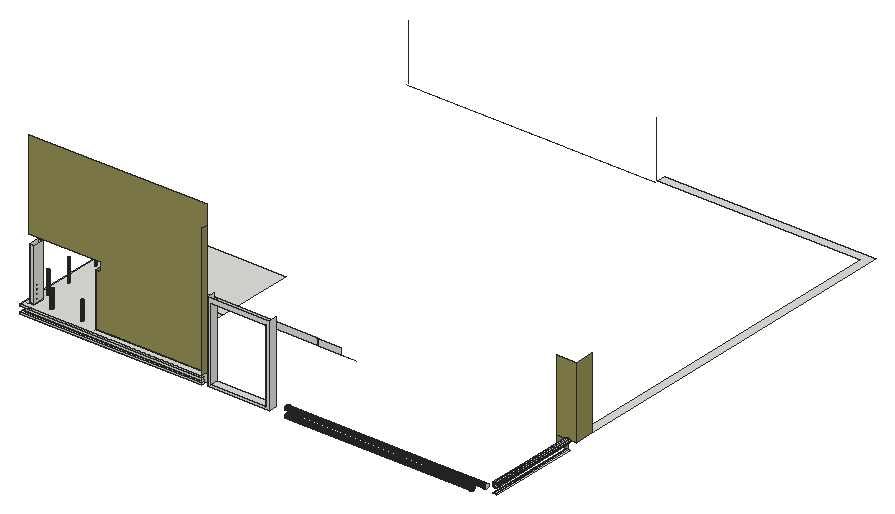
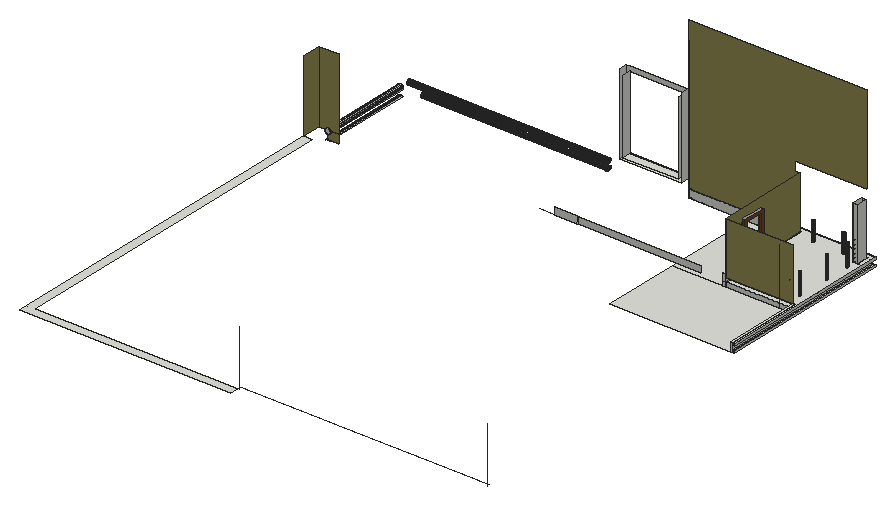
# SketchUp Ruby script. Lengths in inches.
U = 1.inch
M = Sketchup.active_model
def pt(a) = Geom::Point3d.new(a.map { |v| v * U })
def face(e, loops, mat)
  f = e.add_face(loops[0].map { |a| pt(a) })
  loops[1..].each { |l| e.add_face(l.map { |a| pt(a) }).erase! }
  f.material = f.back_material = mat if mat
  f
end
# faces: each face lists its corners as indices into pts; further lists are holes
def faces(e, pts, list, mat = nil) = list.each { |f| face(e, (f[0].is_a?(Array) ? f : [f]).map { |l| l.map { |i| pts[i] } }, mat) }
# xy, xz, yz: faces in a plane at the given z, y or x. An outline is a flat list of corners, or four numbers for a rectangle; further outlines are holes
def ring(l) = l.size == 4 ? [[l[0], l[1]], [l[2], l[1]], [l[2], l[3]], [l[0], l[3]]] : l.each_slice(2).to_a
def flat(e, list, mat, &to3) = list.each { |f| face(e, (f[0].is_a?(Array) ? f : [f]).map { |l| ring(l).map { |u, v| to3.(u, v) } }, mat) }
def xy(e, z, list, mat = nil) = flat(e, list, mat) { |x, y| [x, y, z] }
def xz(e, y, list, mat = nil) = flat(e, list, mat) { |x, z| [x, y, z] }
def yz(e, x, list, mat = nil) = flat(e, list, mat) { |y, z| [x, y, z] }
def lines(e, pts, list) = list.each { |a, b| e.add_line(pt(pts[a]), pt(pts[b])) }
# prism: a flat outline (further loops are holes) pulled along v
def prism(e, loops, v, mat = nil)
  f = face(e, loops, mat); d = Geom::Vector3d.new(v.map { |x| x * U })
  f.pushpull(f.normal.samedirection?(d) ? d.length : -d.length)
end
def box(e, o, s, mat = nil) = prism(e, [[o, [o[0] + s[0], o[1], o[2]], [o[0] + s[0], o[1] + s[1], o[2]], [o[0], o[1] + s[1], o[2]]]], [0, 0, s[2]], mat)
def at(x, y, z, deg = 0) = Geom::Transformation.translation(pt([x, y, z])) * Geom::Transformation.rotation(ORIGIN, Z_AXIS, deg.degrees)
def axes(o, x, y, z) = Geom::Transformation.new([*x, 0, *y, 0, *z, 0, *pt(o).to_a, 1])
def part(name) = M.definitions.add(name)
# library, detail: a bought-in or finely detailed component or shape, given as its bounding box
def library(name, o, s) = part(name).tap { |d| box(d.entities, o, s) }
def detail(e, o, s) = box(e.add_group.entities, o, s)
def put(e, d, t, mat = nil) = e.add_instance(d, t).tap { |i| i.material = mat if mat }
def group(e, t, mat = nil) = e.add_group.tap { |g| g.transformation = t; g.material = mat if mat }.entities
root = M.entities
M.materials.add("[0057_DarkKhaki]").color = [150, 145, 85]
M.materials.add("[0137_Black]").color = [71, 71, 71]
M.materials.add("[Wood Veneer 01]").color = [120, 70, 37]
xy(root,417.65,[[11.875,15.1875,200.79,18.1875],[8.875,18.1875,11.875,116.75],[11.875,18.1875,139.9375,116.75],[8.875,116.75,9.8125,199.5],[9.8125,116.75,11.875,199.5],
  [11.875,116.75,139.9375,199.5]])
xy(root,417.72,[[7.3125,12.1875,7.3125,199.5,9.8125,199.5,9.8125,15.1875,82.85,15.1875,82.85,12.1875],[82.85,12.1875,200.79,15.1875],[9.8125,15.1875,9.8125,116.75,11.875,116.75,11.875,18.1875,82.85,18.1875,82.85,15.1875],[82.85,15.1875,200.79,18.1875],[11.875,18.1875,12.375,21.1875],
  [12.375,18.1875,82.85,21.1875],[11.875,21.1875,12.375,21.75],[12.375,21.1875,82.85,21.75],[11.875,21.75,12.375,116.75],[12.375,21.75,82.85,116.75]])
xy(root,419.53,[[7.3125,12.1875,200.79,12.1875,200.79,15.1875,9.8125,15.1875,9.8125,199.5,7.3125,199.5]])
xy(root,422.78,[[11.875,21.1875,12.375,116.75],[12.375,21.1875,82.85,116.75]])
xy(root,423,[[501.6875,143.77,510.6875,143.77,510.6875,520.875,286.17,520.875,286.17,511.875,501.6875,511.875]])
xy(root,424.77,[[7.1875,12.1875,7.1875,199.5,9.8125,199.5,9.8125,15.1875,200.79,15.1875,200.79,12.1875]])
xy(root,425.13,[[213.98,3.1875,279.92,12.1875]])
xy(root,426.78,[[[7.1875,12.1875,7.1875,199.5,9.8125,199.5,9.8125,116.75,82.85,116.75,82.85,95.21,79.85,95.21,79.85,92.21,82.85,92.21,82.85,73.09,79.85,73.09,79.85,70.09,82.85,70.09,82.85,18.1875,200.79,18.1875,200.79,12.1875,16.875,12.1875,16.875,30.25,9.8125,30.25,9.8125,18.1875,11.9375,18.1875,11.9375,19,16.875,19,16.875,12.1875],[64.82,21.64,65.21,21.69,65.57,21.84,65.88,22.08,66.12,22.39,66.27,22.75,66.32,23.14,66.27,23.53,66.12,23.89,65.88,24.2,65.57,24.44,65.21,24.59,64.82,24.64,64.43,24.59,64.07,24.44,63.76,24.2,63.52,23.89,63.375,23.53,63.32,23.14,63.375,22.75,63.52,22.39,63.76,22.08,64.07,21.84,64.43,21.69],[32.63,21.64,33.02,21.69,33.38,21.84,33.7,22.08,33.93,22.39,34.08,22.75,34.13,23.14,34.08,23.53,33.93,23.89,33.7,24.2,33.38,24.44,33.02,24.59,32.63,24.64,32.25,24.59,31.88,24.44,31.57,24.2,31.34,23.89,31.1875,23.53,31.13,23.14,31.1875,22.75,31.34,22.39,31.57,22.08,31.88,21.84,32.25,21.69],[15.22,38.96,15.47,39,15.69,39.09,15.88,39.24,16.03,39.43,16.125,39.65,16.15,39.89,16.125,40.14,16.03,40.36,15.88,40.55,15.69,40.7,15.47,40.79,15.22,40.82,14.98,40.79,14.76,40.7,14.57,40.55,14.42,40.36,14.33,40.14,14.29,39.89,14.33,39.65,14.42,39.43,14.57,39.24,14.76,39.09,14.98,39],[15.85,101.9,16.09,101.93,16.31,102.03,16.51,102.17,16.66,102.37,16.75,102.59,16.78,102.83,16.75,103.07,16.66,103.3,16.51,103.49,16.31,103.64,16.09,103.73,15.85,103.76,15.61,103.73,15.38,103.64,15.19,103.49,15.04,103.3,14.95,103.07,14.92,102.83,14.95,102.59,15.04,102.37,15.19,102.17,15.38,102.03,15.61,101.93],[15.85,65.84,16.09,65.87,16.31,65.96,16.51,66.11,16.66,66.3,16.75,66.53,16.78,66.77,16.75,67.01,16.66,67.23,16.51,67.43,16.31,67.58,16.09,67.67,15.85,67.7,15.61,67.67,15.38,67.58,15.19,67.43,15.04,67.23,14.95,67.01,14.92,66.77,14.95,66.53,15.04,66.3,15.19,66.11,15.38,65.96,15.61,65.87]],[9.8125,18.1875,11.9375,30.25],[11.9375,19,16.875,30.25],[79.85,70.09,82.85,73.09],[79.85,92.21,82.85,95.21],
  [9.8125,116.75,11.875,199.5]])
xy(root,426.9,[[[7.1875,12.1875,200.79,12.1875,200.79,18.1875,82.85,18.1875,82.85,70.09,79.85,70.09,79.85,73.09,82.85,73.09,82.85,92.21,79.85,92.21,79.85,95.21,82.85,95.21,82.85,116.75,9.8125,116.75,9.8125,199.5,7.1875,199.5],[11.9375,19,16.875,30.25],[64.82,21.64,64.43,21.69,64.07,21.84,63.76,22.08,63.52,22.39,63.375,22.75,63.32,23.14,63.375,23.53,63.52,23.89,63.76,24.2,64.07,24.44,64.43,24.59,64.82,24.64,65.21,24.59,65.57,24.44,65.88,24.2,66.12,23.89,66.27,23.53,66.32,23.14,66.27,22.75,66.12,22.39,65.88,22.08,65.57,21.84,65.21,21.69],[32.63,21.64,32.25,21.69,31.88,21.84,31.57,22.08,31.34,22.39,31.1875,22.75,31.13,23.14,31.1875,23.53,31.34,23.89,31.57,24.2,31.88,24.44,32.25,24.59,32.63,24.64,33.02,24.59,33.38,24.44,33.7,24.2,33.93,23.89,34.08,23.53,34.13,23.14,34.08,22.75,33.93,22.39,33.7,22.08,33.38,21.84,33.02,21.69],[15.22,38.96,14.98,39,14.76,39.09,14.57,39.24,14.42,39.43,14.33,39.65,14.29,39.89,14.33,40.14,14.42,40.36,14.57,40.55,14.76,40.7,14.98,40.79,15.22,40.82,15.47,40.79,15.69,40.7,15.88,40.55,16.03,40.36,16.125,40.14,16.15,39.89,16.125,39.65,16.03,39.43,15.88,39.24,15.69,39.09,15.47,39],[15.85,101.9,15.61,101.93,15.38,102.03,15.19,102.17,15.04,102.37,14.95,102.59,14.92,102.83,14.95,103.07,15.04,103.3,15.19,103.49,15.38,103.64,15.61,103.73,15.85,103.76,16.09,103.73,16.31,103.64,16.51,103.49,16.66,103.3,16.75,103.07,16.78,102.83,16.75,102.59,16.66,102.37,16.51,102.17,16.31,102.03,16.09,101.93],[15.85,65.84,15.61,65.87,15.38,65.96,15.19,66.11,15.04,66.3,14.95,66.53,14.92,66.77,14.95,67.01,15.04,67.23,15.19,67.43,15.38,67.58,15.61,67.67,15.85,67.7,16.09,67.67,16.31,67.58,16.51,67.43,16.66,67.23,16.75,67.01,16.78,66.77,16.75,66.53,16.66,66.3,16.51,66.11,16.31,65.96,16.09,65.87]]])
xy(root,427.53,[[217.11,3.1875,275.76,12.1875]])
xz(root,3.1875,[[[213.98,425.13,279.92,425.13,279.92,510.53,275.76,510.53,275.76,510.5,213.98,510.5],[217.11,427.53,275.76,505.68]]])
xz(root,12.1875,[[7.3125,417.72,200.79,419.53],[7.1875,424.77,200.79,426.78],[7.1875,426.78,16.875,426.9],[16.875,426.78,200.79,426.9]])
xz(root,15.1875,[[9.8125,417.72,200.79,419.53],[9.8125,419.53,200.79,424.77]])
xz(root,18.1875,[[11.875,417.65,200.79,417.72],[82.85,417.72,200.79,426.78],[82.85,426.78,200.79,426.9]])
xz(root,18.1875,[[82.85,426.9,200.79,426.9,200.79,587.24,11.875,587.24,11.875,493.0625,88.41,493.0625,88.41,483,82.85,483]],"[0057_DarkKhaki]")
xz(root,19,[[11.9375,426.78,16.875,426.9],[11.9375,426.9,16.875,483]])
xz(root,21.1875,[[11.875,417.72,12.375,422.78],[12.375,417.72,82.85,422.78]])
xz(root,30.25,[[11.9375,426.78,16.875,426.9],[[11.9375,426.9,16.875,483],[14.9,434.22,15.21,434.26,15.5,434.375,15.74,434.5625,15.93,434.81,16.05,435.1,16.09,435.4,16.05,435.71,15.93,436,15.74,436.24,15.5,436.43,15.21,436.55,14.9,436.59,14.6,436.55,14.3125,436.43,14.07,436.24,13.875,436,13.76,435.71,13.72,435.4,13.76,435.1,13.875,434.81,14.07,434.5625,14.3125,434.375,14.6,434.26],[14.9,438.47,15.21,438.51,15.5,438.625,15.74,438.8125,15.93,439.06,16.05,439.35,16.09,439.65,16.05,439.96,15.93,440.25,15.74,440.49,15.5,440.68,15.21,440.8,14.9,440.84,14.6,440.8,14.3125,440.68,14.07,440.49,13.875,440.25,13.76,439.96,13.72,439.65,13.76,439.35,13.875,439.06,14.07,438.8125,14.3125,438.625,14.6,438.51],[14.9,442.72,15.21,442.76,15.5,442.875,15.74,443.0625,15.93,443.31,16.05,443.6,16.09,443.9,16.05,444.21,15.93,444.5,15.74,444.74,15.5,444.93,15.21,445.05,14.9,445.09,14.6,445.05,14.3125,444.93,14.07,444.74,13.875,444.5,13.76,444.21,13.72,443.9,13.76,443.6,13.875,443.31,14.07,443.0625,14.3125,442.875,14.6,442.76],[14.9,446.97,15.21,447.01,15.5,447.125,15.74,447.3125,15.93,447.56,16.05,447.85,16.09,448.15,16.05,448.46,15.93,448.75,15.74,448.99,15.5,449.18,15.21,449.3,14.9,449.34,14.6,449.3,14.3125,449.18,14.07,448.99,13.875,448.75,13.76,448.46,13.72,448.15,13.76,447.85,13.875,447.56,14.07,447.3125,14.3125,447.125,14.6,447.01],[14.9,429.97,15.21,430.01,15.5,430.125,15.74,430.3125,15.93,430.56,16.05,430.85,16.09,431.15,16.05,431.46,15.93,431.75,15.74,431.99,15.5,432.18,15.21,432.3,14.9,432.34,14.6,432.3,14.3125,432.18,14.07,431.99,13.875,431.75,13.76,431.46,13.72,431.15,13.76,430.85,13.875,430.56,14.07,430.3125,14.3125,430.125,14.6,430.01]]])
xz(root,70.09,[[79.85,426.78,82.85,426.9]])
xz(root,70.09,[[79.85,426.9,82.85,473.09]],"[Wood Veneer 01]")
xz(root,73.09,[[79.85,426.78,82.85,426.9]])
xz(root,73.09,[[79.85,426.9,82.85,470.09]],"[Wood Veneer 01]")
xz(root,92.21,[[79.85,426.78,82.85,426.9]])
xz(root,92.21,[[79.85,426.9,82.85,470.09]],"[Wood Veneer 01]")
xz(root,95.21,[[79.85,426.78,82.85,426.9]])
xz(root,95.21,[[79.85,426.9,82.85,473.09]],"[Wood Veneer 01]")
xz(root,116.75,[[9.8125,417.65,11.875,417.72],[82.85,417.65,86.03,423],[11.875,417.72,12.375,422.78],[12.375,417.72,82.85,422.78],[82.85,423,86.03,429.99],
  [9.8125,426.78,11.875,426.9],[11.875,426.78,82.85,426.9]])
xz(root,116.75,[[[11.875,426.9,82.85,483],[14.9,446.97,14.6,447.01,14.3125,447.125,14.07,447.3125,13.875,447.56,13.76,447.85,13.72,448.15,13.76,448.46,13.875,448.75,14.07,448.99,14.3125,449.18,14.6,449.3,14.9,449.34,15.21,449.3,15.5,449.18,15.74,448.99,15.93,448.75,16.05,448.46,16.09,448.15,16.05,447.85,15.93,447.56,15.74,447.3125,15.5,447.125,15.21,447.01]]],"[0057_DarkKhaki]")
xz(root,122.75,[[500.91,414,501.3,414.05,501.6875,414]])
xz(root,122.75,[[490.125,414,500.91,414,501.3,414.05,501.6875,414,501.6875,423,490.125,423],[490.125,423,510.6875,499.43]],"[0057_DarkKhaki]")
xz(root,123.0625,[[501.3,418.93,500.54,419.03,499.83,419.32,499.22,419.79,498.75,420.4,498.46,421.1,498.36,421.87,498.46,422.625,498.75,423.33,499.22,423.94,499.83,424.41,500.54,424.7,501.3,424.8,502.06,424.7,502.77,424.41,503.375,423.94,503.84,423.33,504.13,422.625,504.23,421.87,504.13,421.1,503.84,420.4,503.375,419.79,502.77,419.32,502.06,419.03]])
xz(root,199.5,[[9.8125,417.65,11.875,426.78],[7.3125,417.72,9.8125,419.53],[7.1875,424.77,9.8125,426.78],[7.1875,426.78,9.8125,426.9]])
yz(root,7.1875,[[12.1875,424.77,199.5,426.78],[12.1875,426.78,199.5,426.9]])
yz(root,7.3125,[[12.1875,417.72,199.5,419.53]])
yz(root,9.8125,[[116.75,417.65,199.5,417.72],[15.1875,417.72,116.75,419.53],[116.75,417.72,199.5,419.53],[15.1875,419.53,199.5,424.77],[116.75,424.77,199.5,426.78],
  [116.75,426.78,199.5,426.9]])
yz(root,11.875,[[18.1875,417.65,116.75,417.72],[21.1875,417.72,116.75,422.78]])
yz(root,11.9375,[[19,426.78,30.25,426.9],[19,426.9,30.25,483]])
yz(root,12.375,[[21.1875,417.72,116.75,422.78]])
yz(root,16.875,[[19,426.78,30.25,426.9],[[19,426.9,30.25,483],[22.6,429.27,22.25,429.3125,21.92,429.45,21.63,429.67,21.41,429.96,21.28,430.29,21.23,430.64,21.28,431,21.41,431.33,21.63,431.61,21.92,431.83,22.25,431.97,22.6,432.02,22.96,431.97,23.29,431.83,23.58,431.61,23.8,431.33,23.93,431,23.98,430.64,23.93,430.29,23.8,429.96,23.58,429.67,23.29,429.45,22.96,429.3125],[22.6,433.77,22.25,433.8125,21.92,433.95,21.63,434.17,21.41,434.46,21.28,434.79,21.23,435.14,21.28,435.5,21.41,435.83,21.63,436.11,21.92,436.33,22.25,436.47,22.6,436.52,22.96,436.47,23.29,436.33,23.58,436.11,23.8,435.83,23.93,435.5,23.98,435.14,23.93,434.79,23.8,434.46,23.58,434.17,23.29,433.95,22.96,433.8125],[22.6,438.27,22.25,438.3125,21.92,438.45,21.63,438.67,21.41,438.96,21.28,439.29,21.23,439.64,21.28,440,21.41,440.33,21.63,440.61,21.92,440.83,22.25,440.97,22.6,441.02,22.96,440.97,23.29,440.83,23.58,440.61,23.8,440.33,23.93,440,23.98,439.64,23.93,439.29,23.8,438.96,23.58,438.67,23.29,438.45,22.96,438.3125],[22.6,442.77,22.25,442.8125,21.92,442.95,21.63,443.17,21.41,443.46,21.28,443.79,21.23,444.14,21.28,444.5,21.41,444.83,21.63,445.11,21.92,445.33,22.25,445.47,22.6,445.52,22.96,445.47,23.29,445.33,23.58,445.11,23.8,444.83,23.93,444.5,23.98,444.14,23.93,443.79,23.8,443.46,23.58,443.17,23.29,442.95,22.96,442.8125]]])
yz(root,79.85,[[70.09,426.78,73.09,426.9],[92.21,426.78,95.21,426.9]])
yz(root,79.85,[[70.09,426.9,70.09,473.09,95.21,473.09,95.21,426.9,92.21,426.9,92.21,470.09,73.09,470.09,73.09,426.9]],"[Wood Veneer 01]")
yz(root,82.85,[[18.1875,417.72,21.1875,426.78],[21.1875,417.72,116.75,417.72,116.75,422.78,92.21,422.78,92.21,422.4375,73.09,422.4375,73.09,422.78,21.1875,422.78],[73.09,422.4375,92.21,422.78],[21.1875,422.78,73.09,422.78,73.09,423.55,92.21,423.55,92.21,422.78,116.75,422.78,116.75,426.78,21.1875,426.78],[73.09,422.78,92.21,423.55],
  [18.1875,426.78,21.1875,426.9],[21.1875,426.78,70.09,426.9],[70.09,426.78,73.09,426.78,73.09,470.09,92.21,470.09,92.21,426.78,95.21,426.78,95.21,473.09,70.09,473.09],[73.09,426.78,92.21,426.9],[95.21,426.78,116.75,426.9]])
yz(root,82.85,[[18.1875,426.9,18.1875,483,116.75,483,116.75,426.9,95.21,426.9,95.21,473.09,70.09,473.09,70.09,426.9]],"[0057_DarkKhaki]")
yz(root,82.85,[[73.09,426.9,92.21,430.75]],"[Wood Veneer 01]")
yz(root,200.79,[[12.1875,417.72,15.1875,419.53],[15.1875,417.72,15.1875,424.77,12.1875,424.77,12.1875,426.78,18.1875,426.78,18.1875,417.72],[12.1875,419.53,15.1875,424.77],[12.1875,426.78,18.1875,426.9]])
yz(root,200.79,[[12.1875,426.9,18.1875,567.22]],"[0057_DarkKhaki]")
yz(root,213.98,[[3.1875,425.13,12.1875,510.5]])
yz(root,217.11,[[3.1875,427.53,12.1875,505.68]])
yz(root,275.76,[[3.1875,427.53,12.1875,505.68]])
yz(root,279.92,[[3.1875,425.13,12.1875,510.53]])
yz(root,499.48,[[18.04,421.36,18.63,421.44,19.17,421.66,19.64,422.02,19.99,422.49,20.22,423.03,20.29,423.61,20.22,424.2,19.99,424.74,19.64,425.2,19.17,425.5625,18.63,425.79,18.04,425.86,17.46,425.79,16.92,425.5625,16.45,425.2,16.1,424.74,15.87,424.2,15.79,423.61,15.87,423.03,16.1,422.49,16.45,422.02,16.92,421.66,17.46,421.44]])
yz(root,510.6875,[[122.75,423,143.77,499.43]],"[0057_DarkKhaki]")
p = [[499.22,26.4375,413.19],[499.83,26.4375,413.66],[499.83,122.75,413.66],[499.22,122.75,413.19],[502.77,26.4375,413.66],[503.375,26.4375,413.19],
  [503.375,122.75,413.19],[502.77,122.75,413.66],[500.54,26.4375,413.95],[500.54,122.75,413.95],[502.06,26.4375,413.95],[502.06,122.75,413.95],
  [286.17,16.92,414.16],[286.17,17.46,413.94],[484.5625,17.46,413.94],[484.5625,16.92,414.16],[286.17,18.04,413.86],[484.5625,18.04,413.86],
  [286.17,18.63,413.94],[484.5625,18.63,413.94],[286.17,19.17,414.16],[484.5625,19.17,414.16],[501.3,26.4375,414.05],[501.3,122.75,414.05],
  [500.91,122.75,414],[501.6875,122.75,414],[286.17,16.45,414.52],[484.5625,16.45,414.52],[286.17,19.64,414.52],[484.5625,19.64,414.52],
  [286.17,16.1,414.99],[484.5625,16.1,414.99],[286.17,19.99,414.99],[484.5625,19.99,414.99],[286.17,15.87,415.53],[484.5625,15.87,415.53],
  [286.17,20.22,415.53],[484.5625,20.22,415.53],[286.17,15.79,416.11],[484.5625,15.79,416.11],[286.17,20.29,416.11],[484.5625,20.29,416.11],
  [286.17,15.87,416.7],[484.5625,15.87,416.7],[286.17,20.22,416.7],[484.5625,20.22,416.7],[286.17,16.1,417.24],[484.5625,16.1,417.24],
  [286.17,19.99,417.24],[484.5625,19.99,417.24],[286.17,16.45,417.7],[484.5625,16.45,417.7],[286.17,19.64,417.7],[484.5625,19.64,417.7],
  [286.17,16.92,418.0625],[484.5625,16.92,418.0625],[286.17,19.17,418.0625],[484.5625,19.17,418.0625],[286.17,17.46,418.29],[484.5625,17.46,418.29],
  [286.17,18.63,418.29],[484.5625,18.63,418.29],[286.17,18.04,418.36],[484.5625,18.04,418.36],[501.3,26.4375,418.93],[500.54,26.4375,419.03],
  [500.54,123.0625,419.03],[501.3,123.0625,418.93],[502.06,26.4375,419.03],[502.06,123.0625,419.03],[499.83,26.4375,419.32],[499.83,123.0625,419.32],
  [502.77,26.4375,419.32],[502.77,123.0625,419.32],[499.22,26.4375,419.79],[499.22,123.0625,419.79],[503.375,26.4375,419.79],[503.375,123.0625,419.79],
  [498.75,26.4375,420.4],[498.75,123.0625,420.4],[503.84,26.4375,420.4],[503.84,123.0625,420.4],[498.46,26.4375,421.1],[498.46,123.0625,421.1],
  [504.13,26.4375,421.1],[504.13,123.0625,421.1],[498.36,26.4375,421.87],[498.36,123.0625,421.87],[504.23,26.4375,421.87],[504.23,123.0625,421.87],
  [286.17,16.92,421.66],[286.17,17.46,421.44],[499.48,17.46,421.44],[499.48,16.92,421.66],[286.17,18.04,421.36],[499.48,18.04,421.36],
  [286.17,18.63,421.44],[499.48,18.63,421.44],[286.17,19.17,421.66],[499.48,19.17,421.66],[286.17,16.45,422.02],[499.48,16.45,422.02],
  [286.17,19.64,422.02],[499.48,19.64,422.02],[498.46,26.4375,422.625],[498.46,123.0625,422.625],[504.13,26.4375,422.625],[504.13,123.0625,422.625],
  [286.17,16.1,422.49],[499.48,16.1,422.49],[286.17,19.99,422.49],[499.48,19.99,422.49],[286.17,15.87,423.03],[499.48,15.87,423.03],
  [286.17,20.22,423.03],[499.48,20.22,423.03],[498.75,26.4375,423.33],[498.75,123.0625,423.33],[503.84,26.4375,423.33],[503.84,123.0625,423.33],
  [286.17,15.79,423.61],[499.48,15.79,423.61],[286.17,20.29,423.61],[499.48,20.29,423.61],[264.92,116.9375,423],[240.73,117.16,423],
  [240.73,117.16,429.99],[264.92,116.9375,429.99],[108.67,118.38,429.99],[238.67,117.18,429.99],[238.67,117.18,423],[108.67,118.38,423],
  [499.22,26.4375,423.94],[499.22,123.0625,423.94],[503.375,26.4375,423.94],[503.375,123.0625,423.94],[286.17,15.87,424.2],[499.48,15.87,424.2],
  [286.17,20.22,424.2],[499.48,20.22,424.2],[499.83,26.4375,424.41],[499.83,123.0625,424.41],[502.77,26.4375,424.41],[502.77,123.0625,424.41],
  [286.17,16.1,424.74],[499.48,16.1,424.74],[286.17,19.99,424.74],[499.48,19.99,424.74],[500.54,26.4375,424.7],[500.54,123.0625,424.7],
  [502.06,26.4375,424.7],[502.06,123.0625,424.7],[286.17,16.45,425.2],[499.48,16.45,425.2],[286.17,19.64,425.2],[499.48,19.64,425.2],
  [501.3,26.4375,424.8],[501.3,123.0625,424.8],[286.17,16.92,425.5625],[499.48,16.92,425.5625],[286.17,19.17,425.5625],[499.48,19.17,425.5625],
  [286.17,17.46,425.79],[499.48,17.46,425.79],[286.17,18.63,425.79],[499.48,18.63,425.79],[286.17,18.04,425.86],[499.48,18.04,425.86],
  [32.25,21.69,426.78],[32.63,21.64,426.78],[32.63,21.64,426.9],[32.25,21.69,426.9],[33.02,21.69,426.78],[33.02,21.69,426.9],
  [64.43,21.69,426.78],[64.82,21.64,426.78],[64.82,21.64,426.9],[64.43,21.69,426.9],[65.21,21.69,426.78],[65.21,21.69,426.9],
  [31.88,21.84,426.78],[31.88,21.84,426.9],[33.38,21.84,426.78],[33.38,21.84,426.9],[64.07,21.84,426.78],[64.07,21.84,426.9],
  [65.57,21.84,426.78],[65.57,21.84,426.9],[31.57,22.08,426.78],[31.57,22.08,426.9],[33.7,22.08,426.78],[33.7,22.08,426.9],
  [63.76,22.08,426.78],[63.76,22.08,426.9],[65.88,22.08,426.78],[65.88,22.08,426.9],[31.34,22.39,426.78],[31.34,22.39,426.9],
  [33.93,22.39,426.78],[33.93,22.39,426.9],[63.52,22.39,426.78],[63.52,22.39,426.9],[66.12,22.39,426.78],[66.12,22.39,426.9],
  [31.1875,22.75,426.78],[31.1875,22.75,426.9],[34.08,22.75,426.78],[34.08,22.75,426.9],[63.375,22.75,426.78],[63.375,22.75,426.9],
  [66.27,22.75,426.78],[66.27,22.75,426.9],[31.13,23.14,426.78],[31.13,23.14,426.9],[34.13,23.14,426.78],[34.13,23.14,426.9],
  [63.32,23.14,426.78],[63.32,23.14,426.9],[66.32,23.14,426.78],[66.32,23.14,426.9],[31.1875,23.53,426.78],[31.1875,23.53,426.9],
  [34.08,23.53,426.78],[34.08,23.53,426.9],[63.375,23.53,426.78],[63.375,23.53,426.9],[66.27,23.53,426.78],[66.27,23.53,426.9],
  [31.34,23.89,426.78],[31.34,23.89,426.9],[33.93,23.89,426.78],[33.93,23.89,426.9],[63.52,23.89,426.78],[63.52,23.89,426.9],
  [66.12,23.89,426.78],[66.12,23.89,426.9],[31.57,24.2,426.78],[31.57,24.2,426.9],[33.7,24.2,426.78],[33.7,24.2,426.9],
  [63.76,24.2,426.78],[63.76,24.2,426.9],[65.88,24.2,426.78],[65.88,24.2,426.9],[31.88,24.44,426.78],[31.88,24.44,426.9],
  [33.38,24.44,426.78],[33.38,24.44,426.9],[64.07,24.44,426.78],[64.07,24.44,426.9],[65.57,24.44,426.78],[65.57,24.44,426.9],
  [32.25,24.59,426.78],[32.25,24.59,426.9],[33.02,24.59,426.78],[33.02,24.59,426.9],[64.43,24.59,426.78],[64.43,24.59,426.9],
  [65.21,24.59,426.78],[65.21,24.59,426.9],[32.63,24.64,426.78],[32.63,24.64,426.9],[64.82,24.64,426.78],[64.82,24.64,426.9],
  [14.76,39.09,426.78],[14.98,39,426.78],[14.98,39,426.9],[14.76,39.09,426.9],[15.22,38.96,426.78],[15.22,38.96,426.9],
  [15.47,39,426.78],[15.47,39,426.9],[15.69,39.09,426.78],[15.69,39.09,426.9],[14.57,39.24,426.78],[14.57,39.24,426.9],
  [15.88,39.24,426.78],[15.88,39.24,426.9],[14.42,39.43,426.78],[14.42,39.43,426.9],[16.03,39.43,426.78],[16.03,39.43,426.9],
  [14.33,39.65,426.78],[14.33,39.65,426.9],[16.125,39.65,426.78],[16.125,39.65,426.9],[14.29,39.89,426.78],[14.29,39.89,426.9],
  [16.15,39.89,426.78],[16.15,39.89,426.9],[14.33,40.14,426.78],[14.33,40.14,426.9],[16.125,40.14,426.78],[16.125,40.14,426.9],
  [14.42,40.36,426.78],[14.42,40.36,426.9],[16.03,40.36,426.78],[16.03,40.36,426.9],[14.57,40.55,426.78],[14.57,40.55,426.9],
  [15.88,40.55,426.78],[15.88,40.55,426.9],[14.76,40.7,426.78],[14.76,40.7,426.9],[15.69,40.7,426.78],[15.69,40.7,426.9],
  [14.98,40.79,426.78],[14.98,40.79,426.9],[15.47,40.79,426.78],[15.47,40.79,426.9],[15.22,40.82,426.78],[15.22,40.82,426.9],
  [15.61,65.87,426.78],[15.85,65.84,426.78],[15.85,65.84,426.9],[15.61,65.87,426.9],[16.09,65.87,426.78],[16.09,65.87,426.9],
  [15.38,65.96,426.78],[15.38,65.96,426.9],[16.31,65.96,426.78],[16.31,65.96,426.9],[15.19,66.11,426.78],[15.19,66.11,426.9],
  [16.51,66.11,426.78],[16.51,66.11,426.9],[15.04,66.3,426.78],[15.04,66.3,426.9],[16.66,66.3,426.78],[16.66,66.3,426.9],
  [14.95,66.53,426.78],[14.95,66.53,426.9],[16.75,66.53,426.78],[16.75,66.53,426.9],[14.92,66.77,426.78],[14.92,66.77,426.9],
  [16.78,66.77,426.78],[16.78,66.77,426.9],[14.95,67.01,426.78],[14.95,67.01,426.9],[16.75,67.01,426.78],[16.75,67.01,426.9],
  [15.04,67.23,426.78],[15.04,67.23,426.9],[16.66,67.23,426.78],[16.66,67.23,426.9],[15.19,67.43,426.78],[15.19,67.43,426.9],
  [16.51,67.43,426.78],[16.51,67.43,426.9],[15.38,67.58,426.78],[15.38,67.58,426.9],[16.31,67.58,426.78],[16.31,67.58,426.9],
  [15.61,67.67,426.78],[15.61,67.67,426.9],[16.09,67.67,426.78],[16.09,67.67,426.9],[15.85,67.7,426.78],[15.85,67.7,426.9],
  [15.38,102.03,426.78],[15.61,101.93,426.78],[15.61,101.93,426.9],[15.38,102.03,426.9],[15.85,101.9,426.78],[15.85,101.9,426.9],
  [16.09,101.93,426.78],[16.09,101.93,426.9],[16.31,102.03,426.78],[16.31,102.03,426.9],[15.19,102.17,426.78],[15.19,102.17,426.9],
  [16.51,102.17,426.78],[16.51,102.17,426.9],[15.04,102.37,426.78],[15.04,102.37,426.9],[16.66,102.37,426.78],[16.66,102.37,426.9],
  [14.95,102.59,426.78],[14.95,102.59,426.9],[16.75,102.59,426.78],[16.75,102.59,426.9],[14.92,102.83,426.78],[14.92,102.83,426.9],
  [16.78,102.83,426.78],[16.78,102.83,426.9],[14.95,103.07,426.78],[14.95,103.07,426.9],[16.75,103.07,426.78],[16.75,103.07,426.9],
  [15.04,103.3,426.78],[15.04,103.3,426.9],[16.66,103.3,426.78],[16.66,103.3,426.9],[15.19,103.49,426.78],[15.19,103.49,426.9],
  [16.51,103.49,426.78],[16.51,103.49,426.9],[15.38,103.64,426.78],[15.38,103.64,426.9],[16.31,103.64,426.78],[16.31,103.64,426.9],
  [15.61,103.73,426.78],[15.61,103.73,426.9],[16.09,103.73,426.78],[16.09,103.73,426.9],[15.85,103.76,426.78],[15.85,103.76,426.9],
  [32.25,21.69,446.03],[32.63,21.64,446.03],[33.02,21.69,446.03],[64.43,21.69,446.03],[64.82,21.64,446.03],[65.21,21.69,446.03],
  [31.88,21.84,446.03],[33.38,21.84,446.03],[64.07,21.84,446.03],[65.57,21.84,446.03],[31.57,22.08,446.03],[33.7,22.08,446.03],
  [63.76,22.08,446.03],[65.88,22.08,446.03],[31.34,22.39,446.03],[33.93,22.39,446.03],[63.52,22.39,446.03],[66.12,22.39,446.03],
  [31.1875,22.75,446.03],[34.08,22.75,446.03],[63.375,22.75,446.03],[66.27,22.75,446.03],[31.13,23.14,446.03],[34.13,23.14,446.03],
  [63.32,23.14,446.03],[66.32,23.14,446.03],[31.1875,23.53,446.03],[34.08,23.53,446.03],[63.375,23.53,446.03],[66.27,23.53,446.03],
  [31.34,23.89,446.03],[33.93,23.89,446.03],[63.52,23.89,446.03],[66.12,23.89,446.03],[31.57,24.2,446.03],[33.7,24.2,446.03],
  [63.76,24.2,446.03],[65.88,24.2,446.03],[31.88,24.44,446.03],[33.38,24.44,446.03],[64.07,24.44,446.03],[65.57,24.44,446.03],
  [32.25,24.59,446.03],[33.02,24.59,446.03],[64.43,24.59,446.03],[65.21,24.59,446.03],[32.63,24.64,446.03],[64.82,24.64,446.03],
  [14.76,39.09,450.4],[14.98,39,450.4],[15.22,38.96,450.4],[15.47,39,450.4],[15.69,39.09,450.4],[14.57,39.24,450.4],
  [15.88,39.24,450.4],[14.42,39.43,450.4],[16.03,39.43,450.4],[14.33,39.65,450.4],[16.125,39.65,450.4],[14.29,39.89,450.4],
  [16.15,39.89,450.4],[14.33,40.14,450.4],[16.125,40.14,450.4],[14.42,40.36,450.4],[16.03,40.36,450.4],[14.57,40.55,450.4],
  [15.88,40.55,450.4],[14.76,40.7,450.4],[15.69,40.7,450.4],[14.98,40.79,450.4],[15.47,40.79,450.4],[15.22,40.82,450.4],
  [15.61,65.87,450.4],[15.85,65.84,450.4],[16.09,65.87,450.4],[15.38,65.96,450.4],[16.31,65.96,450.4],[15.19,66.11,450.4],
  [16.51,66.11,450.4],[15.04,66.3,450.4],[16.66,66.3,450.4],[14.95,66.53,450.4],[16.75,66.53,450.4],[14.92,66.77,450.4],
  [16.78,66.77,450.4],[14.95,67.01,450.4],[16.75,67.01,450.4],[15.04,67.23,450.4],[16.66,67.23,450.4],[15.19,67.43,450.4],
  [16.51,67.43,450.4],[15.38,67.58,450.4],[16.31,67.58,450.4],[15.61,67.67,450.4],[16.09,67.67,450.4],[15.85,67.7,450.4],
  [15.38,102.03,450.4],[15.61,101.93,450.4],[15.85,101.9,450.4],[16.09,101.93,450.4],[16.31,102.03,450.4],[15.19,102.17,450.4],
  [16.51,102.17,450.4],[15.04,102.37,450.4],[16.66,102.37,450.4],[14.95,102.59,450.4],[16.75,102.59,450.4],[14.92,102.83,450.4],
  [16.78,102.83,450.4],[14.95,103.07,450.4],[16.75,103.07,450.4],[15.04,103.3,450.4],[16.66,103.3,450.4],[15.19,103.49,450.4],
  [16.51,103.49,450.4],[15.38,103.64,450.4],[16.31,103.64,450.4],[15.61,103.73,450.4],[16.09,103.73,450.4],[15.85,103.76,450.4],
  [20.875,122.75,423],[20.875,122.75,483],[20.875,511.875,423],[20.875,511.875,483],[509.75,511.875,423],[509.9375,511.875,423],
  [281.04,116.79,423],[284.05,511.875,423],[284.05,511.875,483],[82.85,16.6875,417.72],[82.85,16.6875,426.78],[11.875,16.6875,417.72],
  [11.875,16.6875,426.78],[20.875,508.3125,423],[286.17,508.3125,423],[11.875,116.75,422.78],[9.8125,116.75,422.78],[9.8125,18.1875,426.78],
  [9.8125,18.1875,426.9],[11.9375,18.1875,426.78],[11.9375,18.1875,426.9],[9.8125,30.25,426.78],[9.8125,30.25,426.9]]
faces(root,p,[[0,1,2,3],[4,5,6,7],[1,8,9,2],[10,4,7,11],[8,22,23,24,9],[22,10,11,25,23],[64,65,66,67],[68,64,67,69],
  [65,70,71,66],[72,68,69,73],[70,74,75,71],[76,72,73,77],[74,78,79,75],[80,76,77,81],[78,82,83,79],[84,80,81,85],
  [82,86,87,83],[88,84,85,89],[86,104,105,87],[106,88,89,107],[104,116,117,105],[118,106,107,119],[124,125,126,127],[128,129,130,131],
  [129,126,125,130],[116,132,133,117],[134,118,119,135],[132,140,141,133],[142,134,135,143],[140,148,149,141],[150,142,143,151],[148,156,157,149],
  [156,150,151,157],[168,169,170,171],[169,172,173,170],[174,175,176,177],[175,178,179,176],[180,168,171,181],[172,182,183,173],[184,174,177,185],
  [178,186,187,179],[188,180,181,189],[182,190,191,183],[192,184,185,193],[186,194,195,187],[196,188,189,197],[190,198,199,191],[200,192,193,201],
  [194,202,203,195],[204,196,197,205],[198,206,207,199],[208,200,201,209],[202,210,211,203],[212,204,205,213],[206,214,215,207],[216,208,209,217],
  [210,218,219,211],[220,212,213,221],[214,222,223,215],[224,216,217,225],[218,226,227,219],[228,220,221,229],[222,230,231,223],[232,224,225,233],
  [226,234,235,227],[236,228,229,237],[230,238,239,231],[240,232,233,241],[234,242,243,235],[244,236,237,245],[238,246,247,239],[248,240,241,249],
  [242,250,251,243],[252,244,245,253],[246,254,255,247],[256,248,249,257],[250,258,259,251],[260,252,253,261],[254,260,261,255],[262,256,257,263],
  [258,262,263,259],[264,265,266,267],[265,268,269,266],[268,270,271,269],[270,272,273,271],[274,264,267,275],[272,276,277,273],[278,274,275,279],
  [276,280,281,277],[282,278,279,283],[280,284,285,281],[286,282,283,287],[284,288,289,285],[290,286,287,291],[288,292,293,289],[294,290,291,295],
  [292,296,297,293],[298,294,295,299],[296,300,301,297],[302,298,299,303],[300,304,305,301],[306,302,303,307],[304,308,309,305],[310,306,307,311],
  [308,310,311,309],[312,313,314,315],[313,316,317,314],[318,312,315,319],[316,320,321,317],[322,318,319,323],[320,324,325,321],[326,322,323,327],
  [324,328,329,325],[330,326,327,331],[328,332,333,329],[334,330,331,335],[332,336,337,333],[338,334,335,339],[336,340,341,337],[342,338,339,343],
  [340,344,345,341],[346,342,343,347],[344,348,349,345],[350,346,347,351],[348,352,353,349],[354,350,351,355],[352,356,357,353],[358,354,355,359],
  [356,358,359,357],[360,361,362,363],[361,364,365,362],[364,366,367,365],[366,368,369,367],[370,360,363,371],[368,372,373,369],[374,370,371,375],
  [372,376,377,373],[378,374,375,379],[376,380,381,377],[382,378,379,383],[380,384,385,381],[386,382,383,387],[384,388,389,385],[390,386,387,391],
  [388,392,393,389],[394,390,391,395],[392,396,397,393],[398,394,395,399],[396,400,401,397],[402,398,399,403],[400,404,405,401],[406,402,403,407],
  [404,406,407,405]])
faces(root,p,[[12,13,14,15],[13,16,17,14],[16,18,19,17],[18,20,21,19],[26,12,15,27],[20,28,29,21],[30,26,27,31],[28,32,33,29],
  [34,30,31,35],[32,36,37,33],[38,34,35,39],[36,40,41,37],[42,38,39,43],[40,44,45,41],[46,42,43,47],[44,48,49,45],
  [50,46,47,51],[48,52,53,49],[54,50,51,55],[52,56,57,53],[58,54,55,59],[56,60,61,57],[62,58,59,63],[60,62,63,61],
  [90,91,92,93],[91,94,95,92],[94,96,97,95],[96,98,99,97],[100,90,93,101],[98,102,103,99],[108,100,101,109],[102,110,111,103],
  [112,108,109,113],[110,114,115,111],[120,112,113,121],[114,122,123,115],[136,120,121,137],[122,138,139,123],[144,136,137,145],[138,146,147,139],
  [152,144,145,153],[146,154,155,147],[158,152,153,159],[154,160,161,155],[162,158,159,163],[160,164,165,161],[166,162,163,167],[164,166,167,165],
  [408,171,170,409],[409,170,173,410],[411,177,176,412],[412,176,179,413],[414,181,171,408],[410,173,183,415],[416,185,177,411],[413,179,187,417],
  [418,189,181,414],[415,183,191,419],[420,193,185,416],[417,187,195,421],[422,197,189,418],[419,191,199,423],[424,201,193,420],[421,195,203,425],
  [426,205,197,422],[423,199,207,427],[428,209,201,424],[425,203,211,429],[430,213,205,426],[427,207,215,431],[432,217,209,428],[429,211,219,433],
  [434,221,213,430],[431,215,223,435],[436,225,217,432],[433,219,227,437],[438,229,221,434],[435,223,231,439],[440,233,225,436],[437,227,235,441],
  [442,237,229,438],[439,231,239,443],[444,241,233,440],[441,235,243,445],[446,245,237,442],[443,239,247,447],[448,249,241,444],[445,243,251,449],
  [450,253,245,446],[447,247,255,451],[452,257,249,448],[449,251,259,453],[454,261,253,450],[451,255,261,454],[455,263,257,452],[453,259,263,455],
  [456,267,266,457],[457,266,269,458],[458,269,271,459],[459,271,273,460],[461,275,267,456],[460,273,277,462],[463,279,275,461],[462,277,281,464],
  [465,283,279,463],[464,281,285,466],[467,287,283,465],[466,285,289,468],[469,291,287,467],[468,289,293,470],[471,295,291,469],[470,293,297,472],
  [473,299,295,471],[472,297,301,474],[475,303,299,473],[474,301,305,476],[477,307,303,475],[476,305,309,478],[479,311,307,477],[478,309,311,479],
  [480,315,314,481],[481,314,317,482],[483,319,315,480],[482,317,321,484],[485,323,319,483],[484,321,325,486],[487,327,323,485],[486,325,329,488],
  [489,331,327,487],[488,329,333,490],[491,335,331,489],[490,333,337,492],[493,339,335,491],[492,337,341,494],[495,343,339,493],[494,341,345,496],
  [497,347,343,495],[496,345,349,498],[499,351,347,497],[498,349,353,500],[501,355,351,499],[500,353,357,502],[503,359,355,501],[502,357,359,503],
  [504,363,362,505],[505,362,365,506],[506,365,367,507],[507,367,369,508],[509,371,363,504],[508,369,373,510],[511,375,371,509],[510,373,377,512],
  [513,379,375,511],[512,377,381,514],[515,383,379,513],[514,381,385,516],[517,387,383,515],[516,385,389,518],[519,391,387,517],[518,389,393,520],
  [521,395,391,519],[520,393,397,522],[523,399,395,521],[522,397,401,524],[525,403,399,523],[524,401,405,526],[527,407,403,525],[526,405,407,527]],"[0137_Black]")
lines(root,p,[[528,529],[530,531],[532,533],[534,124],[535,536],[537,538],[539,540],[541,542],[543,544],[545,546],[547,548],[549,550]])
